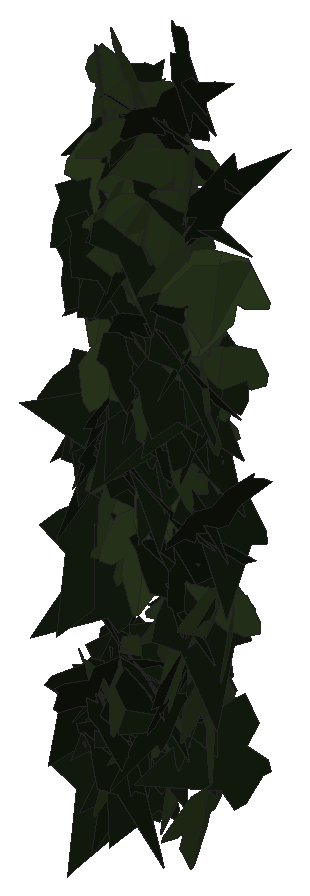
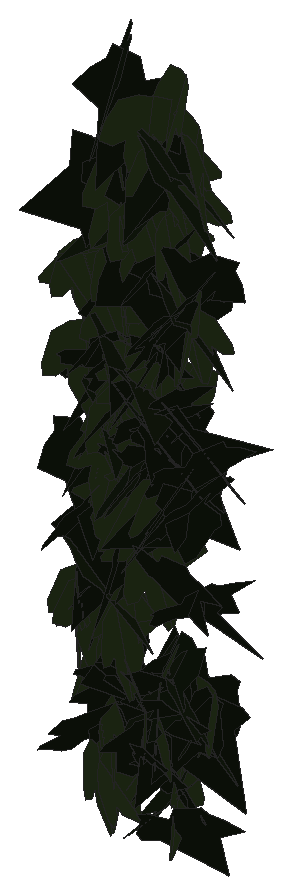
# SketchUp Ruby script. Lengths in inches.
U = 1.inch
M = Sketchup.active_model
def pt(a) = Geom::Point3d.new(a.map { |v| v * U })
def face(e, loops, mat)
  f = e.add_face(loops[0].map { |a| pt(a) })
  loops[1..].each { |l| e.add_face(l.map { |a| pt(a) }).erase! }
  f.material = f.back_material = mat if mat
  f
end
# faces: each face lists its corners as indices into pts; further lists are holes
def faces(e, pts, list, mat = nil) = list.each { |f| face(e, (f[0].is_a?(Array) ? f : [f]).map { |l| l.map { |i| pts[i] } }, mat) }
# xy, xz, yz: faces in a plane at the given z, y or x. An outline is a flat list of corners, or four numbers for a rectangle; further outlines are holes
def ring(l) = l.size == 4 ? [[l[0], l[1]], [l[2], l[1]], [l[2], l[3]], [l[0], l[3]]] : l.each_slice(2).to_a
def flat(e, list, mat, &to3) = list.each { |f| face(e, (f[0].is_a?(Array) ? f : [f]).map { |l| ring(l).map { |u, v| to3.(u, v) } }, mat) }
def xy(e, z, list, mat = nil) = flat(e, list, mat) { |x, y| [x, y, z] }
def xz(e, y, list, mat = nil) = flat(e, list, mat) { |x, z| [x, y, z] }
def yz(e, x, list, mat = nil) = flat(e, list, mat) { |y, z| [x, y, z] }
def lines(e, pts, list) = list.each { |a, b| e.add_line(pt(pts[a]), pt(pts[b])) }
# prism: a flat outline (further loops are holes) pulled along v
def prism(e, loops, v, mat = nil)
  f = face(e, loops, mat); d = Geom::Vector3d.new(v.map { |x| x * U })
  f.pushpull(f.normal.samedirection?(d) ? d.length : -d.length)
end
def box(e, o, s, mat = nil) = prism(e, [[o, [o[0] + s[0], o[1], o[2]], [o[0] + s[0], o[1] + s[1], o[2]], [o[0], o[1] + s[1], o[2]]]], [0, 0, s[2]], mat)
def at(x, y, z, deg = 0) = Geom::Transformation.translation(pt([x, y, z])) * Geom::Transformation.rotation(ORIGIN, Z_AXIS, deg.degrees)
def axes(o, x, y, z) = Geom::Transformation.new([*x, 0, *y, 0, *z, 0, *pt(o).to_a, 1])
def part(name) = M.definitions.add(name)
# library, detail: a bought-in or finely detailed component or shape, given as its bounding box
def library(name, o, s) = part(name).tap { |d| box(d.entities, o, s) }
def detail(e, o, s) = box(e.add_group.entities, o, s)
def put(e, d, t, mat = nil) = e.add_instance(d, t).tap { |i| i.material = mat if mat }
def group(e, t, mat = nil) = e.add_group.tap { |g| g.transformation = t; g.material = mat if mat }.entities
root = M.entities
M.materials.add("efeu1").color = [18, 25, 13]
M.materials.add("efeu2").color = [43, 57, 29]
c1 = part("ivyleaf_9")
p = [[1.54,2.16,1.25],[1.36,2.04,1.19],[-0.21,0.99,0.68],[-0.71,1.11,0.82],[-0.85,0.86,0.67],[-0.8,0.17,0.21],
  [-0.9,-0.01,0.1],[-0.67,-0.16,-0.02],[-0.08,-0.08,-0.05],[-0.03,-0.6,-0.4],[0.65,-0.88,-0.66],[0.83,-0.6,-0.49],
  [1.29,-0.42,-0.43],[1.8125,-0.07,-0.26],[1.21,0.44,0.15]]
faces(c1.entities,p,[[0,1,2,3,4,5,6,7,8,9,10,11,12,13,14]],"efeu1")
c2 = part("ivyleaf_10")
p = [[0,0.5,-0.03],[-0.0625,2.02,-0.43],[-0.19,2.01,-0.46],[-0.54,1.05,-0.29],[-0.52,0.625,-0.18],[-0.83,0.76,-0.28],
  [-1.16,0.64,-0.33],[-1.15,0.33,-0.24],[-0.77,-0.39,0.02],[-0.3,-0.51,0.16],[0.04,-0.48,0.23],[-0.02,2.01,-0.4375],
  [-0.06,2.01,-0.43],[0.04,-0.49,0.23],[0.67,-0.49,0.14],[1.38,0.36,-0.2],[1.375,0.51,-0.24],[0.81,0.65,-0.19],
  [0.62,0.59,-0.15],[0.6,1.09,-0.28],[0.5,1.23,-0.31]]
faces(c2.entities,p,[[0,1,2,3,4,5,6,7,8,9,10],[11,12,0,13,14,15,16,17,18,19,20]],"efeu2")
put(root,c1,axes([31.97,223.8125,224.56],[0.09124,0.25938,-0.41761],[-0.1211,-0.39979,-0.27477],[-0.47645,0.15129,-0.01014]))
put(root,c1,axes([31.76,224.08,228.32],[-0.19188,-0.46171,0.00306],[0.00038,-0.00347,-0.49999],[0.46172,-0.19187,0.00168]))
put(root,c1,axes([32,223.96,224.97],[-0.42402,0.22239,-0.14405],[0.12752,-0.067,-0.4788],[-0.23226,-0.44278,0.0001]))
put(root,c1,axes([31.81,224.0625,226.35],[-0.25772,-0.40985,0.1249],[0.00654,-0.1495,-0.47708],[0.42841,-0.24427,0.08242]))
put(root,c1,axes([31.9,224.19,223.26],[-0.40102,-0.29496,-0.04671],[0.04546,0.017,-0.49764],[0.29515,-0.40337,0.01318]))
put(root,c2,axes([31.85,223.625,224.67],[-0.40011,0.28912,-0.07953],[0.06084,-0.05158,-0.4936],[-0.29362,-0.40466,0.0061]))
put(root,c2,axes([31.94,223.8,232.64],[0.37563,-0.31092,-0.11061],[-0.05857,0.10211,-0.48594],[0.32476,0.37803,0.04029]))
put(root,c2,axes([32.03,223.7,230.36],[-0.3931,0.26949,0.15115],[-0.11897,0.09373,-0.47651],[-0.28517,-0.41059,-0.00957]))
put(root,c1,axes([31.76,224.09,227.77],[0.05876,-0.49556,-0.03113],[0.00034,0.03139,-0.49901],[0.49654,0.05862,0.00402]))
put(root,c1,axes([32.03,224.25,226.89],[-0.45007,-0.11967,-0.18199],[0.18011,0.03042,-0.46544],[0.12247,-0.48451,0.01573]))
put(root,c1,axes([32.03,223.82,227.92],[-0.19506,0.21915,-0.40488],[0.23504,-0.33069,-0.29223],[-0.39586,-0.30433,0.02599]))
put(root,c2,axes([31.95,223.74,232.79],[-0.3885,0.25494,-0.18458],[0.07399,-0.21103,-0.4472],[-0.30593,-0.37479,0.12625]))
put(root,c1,axes([32.27,223.69,226.25],[-0.49705,0.02946,0.04554],[-0.04672,-0.01937,-0.49744],[-0.02754,-0.49876,0.02201]))
put(root,c1,axes([31.86,223.6875,230.39],[0.14981,-0.40054,-0.25908],[-0.09198,0.2422,-0.42764],[0.46808,0.17579,-0.00112]))
put(root,c2,axes([32.08,223.76,223.625],[0.11865,-0.40945,-0.26129],[-0.00161,0.26864,-0.4217],[0.48572,0.1009,0.06243]))
put(root,c2,axes([31.98,223.71,230.2],[0.49718,-0.04443,0.02902],[0.0284,-0.00824,-0.49912],[0.04483,0.49795,-0.00567]))
put(root,c1,axes([31.93,223.83,231.03],[-0.18374,-0.31446,-0.34257],[0.15796,0.30423,-0.364],[0.43736,-0.24198,-0.01246]))
put(root,c1,axes([32.32,223.69,228.6875],[-0.47328,0.15711,-0.03642],[0.0335,-0.01467,-0.49866],[-0.15775,-0.47445,0.00336]))
put(root,c1,axes([32.26,224.23,224.68],[-0.48247,-0.13119,-0.00295],[0.00296,0.00038,-0.49999],[0.13118,-0.48248,0.00041]))
put(root,c1,axes([32.01,223.73,224.69],[0.43491,0.23003,-0.08914],[-0.08025,-0.03892,-0.49198],[-0.23328,0.44224,0.00306]))
put(root,c1,axes([32.07,223.34,224.82],[0.27028,0.41507,0.06833],[0.03321,0.05991,-0.49529],[-0.41934,0.27227,0.00481]))
put(root,c1,axes([32.36,223.59,230.45],[-0.36444,0.3418,-0.01894],[0.01177,-0.01512,-0.49963],[-0.34212,-0.36462,0.00298]))
put(root,c1,axes([32.5,223.71,228.14],[-0.22429,0.00025,0.44687],[-0.44686,0.00393,-0.22428],[-0.00363,-0.49998,-0.00154]))
put(root,c1,axes([31.81,223.78,227.65],[0.47621,-0.05199,0.14324],[0.1449,0.00904,-0.47846],[0.04716,0.49721,0.02367]))
put(root,c1,axes([31.92,223.75,230.57],[0.1841,-0.45831,-0.07782],[-0.00737,0.08081,-0.49337],[0.46482,0.1828,0.023]))
put(root,c1,axes([32.2,223.94,223.79],[-0.43021,0.04534,-0.25072],[0.25126,-0.00607,-0.43224],[-0.04224,-0.4979,-0.01756]))
put(root,c1,axes([32.48,223.63,232.27],[-0.30853,0.38454,0.08331],[-0.0612,0.05767,-0.49288],[-0.38867,-0.31433,0.01148]))
put(root,c1,axes([32.5,223.7,232.48],[-0.40566,0.29065,0.03108],[-0.05185,-0.01924,-0.49693],[-0.28767,-0.40639,0.04575]))
put(root,c1,axes([32.03,223.89,227.84],[0.29444,-0.34357,-0.21276],[-0.11841,0.17834,-0.45186],[0.38638,0.31647,0.02366]))
put(root,c1,axes([32.32,223.69,228.63],[-0.18518,0.33751,-0.31906],[0.14547,-0.28405,-0.38491],[-0.44108,-0.23538,0.00701]))
put(root,c2,axes([32.26,223.77,231.3],[0.06668,-0.49504,-0.02214],[0.00099,0.02247,-0.49949],[0.49553,0.06657,0.00397]))
put(root,c1,axes([32.1,224.25,223.34],[-0.11633,-0.41344,0.256],[0.05804,-0.27315,-0.41475],[0.4828,-0.06678,0.11155]))
put(root,c1,axes([32.45,224.15,223.94],[-0.4985,0.03103,-0.02303],[0.02283,-0.00399,-0.49946],[-0.03118,-0.49902,0.00256]))
put(root,c2,axes([32.05,224.24,224.57],[0.30303,-0.30916,0.25019],[0.25601,-0.08908,-0.42015],[0.30436,0.38273,0.10431]))
put(root,c1,axes([31.9,224.05,225.06],[0.33313,-0.31988,0.19159],[0.14297,-0.1277,-0.46179],[0.34437,0.36245,0.00638]))
put(root,c2,axes([32.28,223.76,227.62],[0.16065,0.43552,-0.18577],[-0.13633,-0.14532,-0.45858],[-0.45344,0.19799,0.07206]))
put(root,c1,axes([32.01,223.8,230.25],[0.20253,-0.3933,-0.23301],[0.00525,0.25684,-0.42896],[0.45711,0.17131,0.10817]))
put(root,c1,axes([32.1,223.48,224.42],[0.40194,-0.19276,-0.22648],[-0.16797,0.16708,-0.44031],[0.24542,0.43003,0.06956]))
put(root,c1,axes([32.04,224.27,224.34],[0.11301,-0.45921,0.16235],[0.0237,-0.16128,-0.47268],[0.48648,0.11453,-0.01469]))
put(root,c2,axes([32.21,223.61,231.8],[0.47878,0.14365,-0.01144],[-0.01023,-0.00569,-0.49986],[-0.14375,0.47889,-0.00251]))
put(root,c2,axes([32.37,223.6875,230.5],[-0.30453,-0.39634,0.01333],[0.03764,-0.04561,-0.49649],[0.39477,-0.30139,0.05761]))
put(root,c1,axes([32.08,223.73,223.69],[0.28701,-0.40942,-0.00119],[-0.00117,0.00064,-0.5],[0.40942,0.28701,-0.00059]))
put(root,c1,axes([32.21,223.77,230.16],[0.07386,-0.4766,-0.13189],[-0.01252,0.13151,-0.48223],[0.49436,0.07453,0.00749]))
put(root,c2,axes([32.41,223.48,233.1875],[-0.3871,0.31615,0.01424],[-0.01337,0.00614,-0.49978],[-0.31619,-0.38731,0.0037]))
put(root,c1,axes([32.54,223.81,230.91],[0.11847,0.39138,-0.28773],[-0.08458,-0.27502,-0.40892],[-0.47834,0.14556,0.00104]))
put(root,c2,axes([32.46,223.87,226.6875],[-0.13966,-0.46718,0.11062],[0.01449,-0.11926,-0.48535],[0.47988,-0.13237,0.04685]))
put(root,c2,axes([32.48,223.58,232.22],[-0.26638,-0.4223,-0.0265],[0.03349,0.01017,-0.49877],[0.42181,-0.2675,0.02287]))
put(root,c1,axes([32.2,224.09,227.36],[0.21269,-0.4508,0.03926],[0.01744,-0.03519,-0.49846],[0.45217,0.21341,0.00075]))
put(root,c1,axes([32.26,224.06,224.43],[0.02189,-0.43523,-0.24515],[0.04758,0.24608,-0.43264],[0.49725,-0.00439,0.05219]))
put(root,c2,axes([32.28,223.48,229.15],[0.22865,0.37839,0.23354],[0.11364,0.20415,-0.44205],[-0.42989,0.25523,0.00736]))
put(root,c2,axes([32.42,223.48,224.98],[0.12674,-0.36146,-0.32138],[0.09571,0.3444,-0.34961],[0.47411,0.0271,0.15649]))
put(root,c2,axes([32.29,224.36,224.8125],[-0.16203,0.0756,-0.46694],[0.21811,-0.42603,-0.14466],[-0.41973,-0.25056,0.10508]))
put(root,c1,axes([32.45,223.99,228.8],[-0.19301,-0.44629,0.11649],[-0.02354,-0.11659,-0.48565],[0.46064,-0.19295,0.024]))
put(root,c2,axes([32.56,223.6875,231.125],[-0.25887,-0.41422,0.10679],[0.00736,-0.12912,-0.48299],[0.4277,-0.24849,0.07295]))
put(root,c1,axes([32.43,223.71,223.98],[0.42151,0.10435,0.24787],[-0.24155,-0.05574,0.43422],[0.11825,-0.4858,0.00342]))
put(root,c2,axes([32.77,223.73,224.42],[-0.4028,0.00107,0.29623],[-0.29327,-0.07206,-0.3985],[0.04184,-0.49478,0.05868]))
put(root,c1,axes([32.85,223.81,228.69],[-0.39199,0.28414,0.12492],[-0.09797,0.07768,-0.48412],[-0.29452,-0.40402,-0.00522]))
put(root,c1,axes([32.78,223.53,228.97],[0.01403,0.38884,0.31401],[-0.18322,0.29627,-0.35869],[-0.46501,-0.105,0.1508]))
put(root,c1,axes([32.34,223.8125,230.95],[0.09412,-0.49105,-0.00307],[-0.0022,0.00271,-0.49999],[0.49106,0.09413,-0.00165]))
put(root,c2,axes([32.64,223.87,231.5],[-0.27755,-0.38706,0.15216],[-0.04114,-0.15648,-0.4731],[0.41385,-0.27513,0.05502]))
put(root,c1,axes([32.58,223.48,232.55],[0.40101,0.21563,-0.20663],[-0.24896,0.0503,-0.43068],[-0.16495,0.4483,0.14771]))
put(root,c1,axes([32.6,223.9,228.53],[-0.28924,-0.37807,0.15299],[-0.01951,-0.17452,-0.46815],[0.40738,-0.27678,0.0862]))
put(root,c1,axes([32.3,224.01,224.9],[0.24205,-0.40372,0.16858],[0.10862,-0.13117,-0.4701],[0.42381,0.2642,0.02421]))
put(root,c1,axes([32.51,223.35,229.59],[0.28052,-0.2027,-0.36086],[-0.19777,0.3173,-0.33197],[0.36359,0.32899,0.09784]))
put(root,c1,axes([32.77,223.85,229.56],[-0.48755,-0.08209,-0.07456],[0.07282,0.01656,-0.49439],[0.08364,-0.49294,-0.00419]))
put(root,c1,axes([32.47,223.93,228.02],[0.06801,-0.49414,0.03465],[0.00363,-0.03448,-0.4988],[0.49534,0.06809,-0.00111]))
put(root,c2,axes([32.62,223.67,226.89],[0.28714,0.40284,-0.0726],[-0.04742,-0.05535,-0.49466],[-0.40657,0.29096,0.00642]))
put(root,c2,axes([32.75,223.61,232.77],[-0.43896,-0.23847,-0.02119],[0.01206,0.02218,-0.49936],[0.23911,-0.43891,-0.01371]))
put(root,c1,axes([32.32,223.71,227.375],[0.31244,-0.22465,0.31923],[0.27667,-0.16101,-0.3841],[0.27538,0.41666,0.0237]))
put(root,c2,axes([32.78,224.12,225.75],[0.02349,-0.49941,-0.00635],[0.00736,0.0067,-0.4999],[0.49939,0.0234,0.00767]))
put(root,c2,axes([32.68,223.68,229.14],[0.23704,0.43794,-0.04491],[-0.01505,-0.04291,-0.49793],[-0.43998,0.23741,-0.00716]))
put(root,c1,axes([32.76,224.09,228.15],[-0.38092,-0.29098,-0.14223],[0.141,0.04869,-0.47723],[0.29158,-0.40368,0.04497]))
put(root,c1,axes([32.625,224.22,225.09],[-0.25057,-0.3508,-0.25329],[0.25551,0.11625,-0.41377],[0.34918,-0.33679,0.12101]))
put(root,c2,axes([32.91,223.7,229.875],[0.45486,-0.00046,-0.2076],[-0.19606,0.16343,-0.42994],[0.06825,0.47254,0.14849]))
put(root,c2,axes([32.78,224.32,223.7],[0.13125,-0.40418,0.26346],[0.08981,-0.2478,-0.42489],[0.47403,0.15886,0.00755]))
put(root,c1,axes([32.54,224.0625,228.05],[0.28103,-0.40376,0.08944],[0.0569,-0.06936,-0.49189],[0.40961,0.28665,0.00696]))
put(root,c2,axes([32.89,223.67,231.46],[0.04687,-0.49777,-0.00482],[-0.00186,0.00467,-0.49997],[0.49779,0.04689,-0.00142]))
put(root,c2,axes([32.92,223.84,229.92],[-0.49177,-0.09022,0.00468],[-0.00207,-0.01465,-0.49978],[0.09032,-0.49157,0.01404]))
put(root,c1,axes([32.47,223.8,232.08],[0.35609,-0.15178,0.31649],[0.2899,-0.12699,-0.38708],[0.19788,0.45917,-0.00244]))
put(root,c1,axes([32.875,223.4,229.94],[0.30797,0.39113,-0.04658],[-0.02401,-0.04038,-0.49779],[-0.39317,0.30884,-0.0061]))
put(root,c1,axes([33.03,223.65,224.8],[-0.42302,0.18105,-0.19565],[0.16524,-0.10985,-0.45894],[-0.20917,-0.45294,0.0331]))
put(root,c2,axes([33,223.72,231.91],[-0.39005,-0.31142,0.02963],[-0.02416,-0.01724,-0.49912],[0.31189,-0.3908,-0.0016]))
put(root,c1,axes([32.6875,223.97,229.09],[0.19151,-0.46156,-0.01708],[0.02884,0.0304,-0.49824],[0.46097,0.18985,0.03826]))
put(root,c2,axes([32.93,224.01,228.22],[-0.37803,-0.31409,-0.09186],[0.11675,0.00167,-0.48618],[0.30571,-0.38903,0.07207]))
put(root,c1,axes([32.75,223.98,224.81],[-0.04185,-0.40929,-0.28413],[0.11021,0.27046,-0.40584],[0.4859,-0.09659,0.06757]))
put(root,c1,axes([33.23,223.6875,229.57],[-0.33201,0.37381,-0.00581],[0.00459,-0.0037,-0.49997],[-0.37383,-0.33204,-0.00097]))
put(root,c2,axes([33.07,223.65,231.39],[-0.25022,-0.4283,0.06283],[-0.00694,-0.0686,-0.49522],[0.43283,-0.2487,0.02839]))
put(root,c2,axes([33.05,223.92,228.62],[-0.10427,-0.48798,0.03165],[0.01315,-0.03515,-0.49859],[0.48883,-0.10314,0.02016]))
put(root,c1,axes([32.74,223.67,226.6],[0.34128,-0.36515,-0.01401],[-0.00377,0.01566,-0.49974],[0.3654,0.3412,0.00793]))
put(root,c1,axes([33.03,223.45,224.83],[0.07125,0.16452,0.46675],[0.13407,0.44751,-0.17821],[-0.47639,0.15055,0.01966]))
put(root,c1,axes([33.1,223.64,226.59],[0.17563,-0.04095,-0.46635],[-0.38796,0.26602,-0.16947],[0.26199,0.42138,0.06167]))
put(root,c2,axes([32.85,223.84,227.49],[0.29039,0.36487,0.18039],[0.1233,0.13232,-0.46614],[-0.3879,0.31521,-0.01312]))
put(root,c1,axes([32.78,223.59,231.57],[0.45713,-0.17882,-0.09516],[-0.01602,0.20223,-0.457],[0.20193,0.42086,0.17916]))
put(root,c2,axes([33.05,223.92,225.9],[-0.21003,0.45002,0.05804],[-0.02864,0.05068,-0.4966],[-0.45284,-0.21192,0.00449]))
put(root,c2,axes([33.13,223.76,230.66],[-0.06327,-0.49463,-0.03661],[0.00059,0.03684,-0.49864],[0.49598,-0.06314,-0.00408]))
put(root,c2,axes([33.1875,223.99,224.36],[0.37535,-0.24685,-0.21951],[-0.11008,0.21979,-0.4354],[0.31145,0.37518,0.11065]))
put(root,c2,axes([33.21,223.51,225.53],[0.30026,-0.36048,-0.17293],[-0.11423,0.1299,-0.46912],[0.38314,0.32122,-0.00435]))
put(root,c1,axes([32.83,223.9375,227.87],[0.30768,-0.38644,0.07742],[0.04334,-0.06444,-0.49393],[0.39173,0.31066,-0.00616]))
put(root,c2,axes([33.1875,224.04,225.97],[-0.39611,-0.305,-0.00825],[0.01808,-0.00996,-0.49957],[0.30458,-0.39607,0.01892]))
put(root,c1,axes([33.46,223.85,226.27],[-0.30681,0.36583,0.14844],[-0.13202,0.0821,-0.47522],[-0.37207,-0.3308,0.04622]))
put(root,c1,axes([33.15,223.24,232.93],[0.22566,0.4411,0.06715],[0.03721,0.05638,-0.49542],[-0.44463,0.22859,-0.00738]))
put(root,c2,axes([33.04,223.48,229.02],[-0.14458,-0.3173,-0.35835],[0.22724,0.28396,-0.34311],[0.42126,-0.26208,0.0621]))
put(root,c2,axes([33.22,223.5625,228.15],[-0.16996,0.33807,0.32684],[-0.13076,0.29985,-0.37815],[-0.45168,-0.21401,-0.01351]))
put(root,c1,axes([33.11,223.65,226.83],[0.40068,0.29264,-0.06184],[-0.04979,-0.03668,-0.49616],[-0.29493,0.40376,-0.00026]))
put(root,c1,axes([33.43,223.54,228.3125],[-0.09607,0.32805,0.3649],[-0.10329,0.34998,-0.34182],[-0.47969,-0.14106,0.00052]))
put(root,c1,axes([33.07,223.94,228.55],[0.2354,-0.37513,-0.2321],[-0.11483,0.2019,-0.44278],[0.42591,0.26176,0.0089]))
put(root,c1,axes([32.83,223.68,229.32],[0.28931,-0.22788,0.33818],[0.27213,-0.20093,-0.3682],[0.30371,0.39711,0.00777]))
put(root,c1,axes([33.24,223.48,233.51],[0.30234,-0.16196,-0.36381],[-0.32865,0.15649,-0.34279],[0.2249,0.44641,-0.01183]))
put(root,c1,axes([33.08,223.54,229.29],[0.20082,-0.3259,-0.32165],[-0.06837,0.32595,-0.37294],[0.45277,0.19377,0.08635]))
put(root,c1,axes([33.36,223.97,229.37],[-0.36411,-0.339,0.05004],[-0.03712,-0.03358,-0.49749],[0.34066,-0.36599,-0.00072]))
put(root,c2,axes([33.38,223.93,226.04],[-0.43318,-0.24442,0.05113],[-0.009,-0.08703,-0.49229],[0.24955,-0.42742,0.071]))
put(root,c2,axes([33.375,223.77,223.49],[0.03893,-0.49807,-0.02026],[0.00114,0.02041,-0.49958],[0.49848,0.03885,0.00272]))
put(root,c1,axes([33.5,224.34,224.01],[-0.32311,-0.18396,0.3343],[-0.19277,-0.29934,-0.35105],[0.3293,-0.35574,0.12252]))
put(root,c1,axes([33.14,223.88,229.69],[0.10667,-0.48791,-0.02374],[0.00141,0.02461,-0.49939],[0.48849,0.10647,0.00663]))
put(root,c2,axes([33.67,223.49,228.93],[-0.16702,0.07511,0.46526],[-0.43806,0.15729,-0.18265],[-0.17379,-0.46864,0.01327]))
put(root,c2,axes([33.36,223.53,232.05],[0.30659,-0.37867,-0.11231],[-0.00055,0.14177,-0.47948],[0.39497,0.29413,0.08651]))
put(root,c2,axes([33.46,223.875,226.11],[0.10454,-0.46366,0.15521],[0.04661,-0.14855,-0.47514],[0.48672,0.11381,0.01216]))
put(root,c2,axes([33.49,223.57,225.15],[0.0055,-0.2968,-0.40234],[0.02521,0.40202,-0.29622],[0.49933,-0.01703,0.01939]))
put(root,c1,axes([33.3,223.85,226.01],[0.05587,-0.49362,-0.0567],[-0.01451,0.05541,-0.49671],[0.49666,0.05714,-0.00814]))
put(root,c1,axes([33.32,224.24,227.28],[0.04672,-0.49492,0.05359],[-0.0038,-0.05418,-0.49704],[0.4978,0.04604,-0.00882]))
put(root,c2,axes([33.59,223.84,229.4],[-0.36309,-0.33792,0.06304],[-0.01273,-0.07842,-0.49365],[0.34351,-0.36009,0.04834]))
put(root,c2,axes([33.47,223.89,230.52],[0.42765,0.24868,-0.07263],[-0.05369,-0.05205,-0.49438],[-0.25344,0.43064,-0.01782]))
put(root,c2,axes([33.58,223.99,225.85],[0.27761,-0.37819,-0.17294],[-0.02762,0.19071,-0.46138],[0.41493,0.26572,0.085]))
put(root,c2,axes([33.61,223.74,230.54],[-0.24518,-0.43271,0.05145],[0.03863,-0.08038,-0.49198],[0.43405,-0.23727,0.07284]))
put(root,c1,axes([33.49,223.6,231.46],[0.12915,0.15983,0.45582],[0.23736,0.38994,-0.20398],[-0.42069,0.26908,0.02485]))
put(root,c1,axes([33.77,223.47,227.68],[0.00898,0.49964,-0.01672],[-0.00016,-0.01672,-0.49972],[-0.49992,0.00898,-0.00014]))
